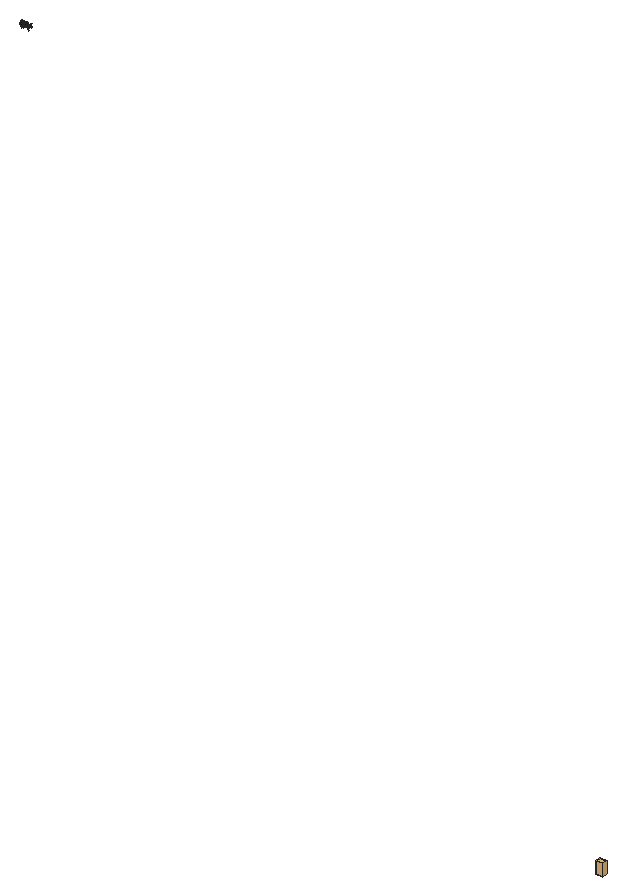
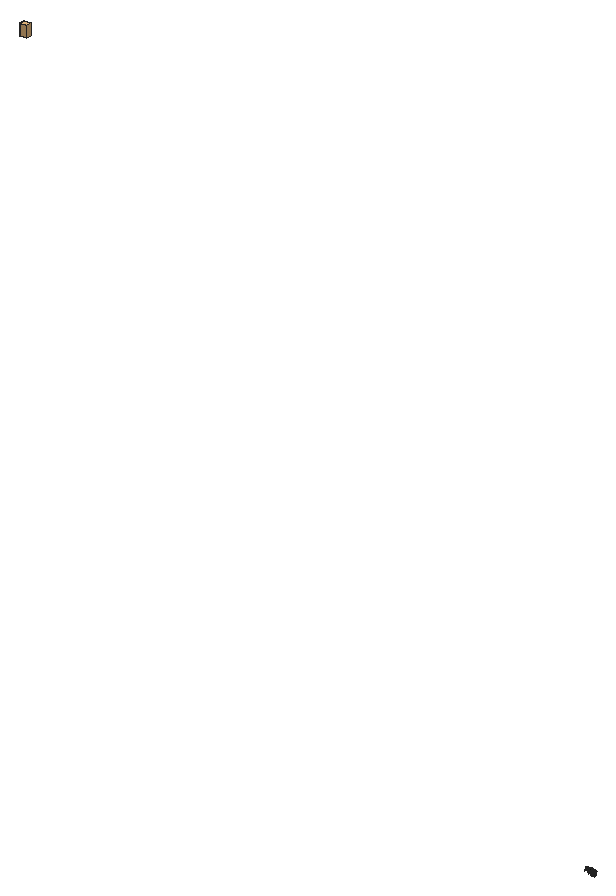
# SketchUp Ruby script. Lengths in inches.
U = 1.inch
M = Sketchup.active_model
def pt(a) = Geom::Point3d.new(a.map { |v| v * U })
def face(e, loops, mat)
  f = e.add_face(loops[0].map { |a| pt(a) })
  loops[1..].each { |l| e.add_face(l.map { |a| pt(a) }).erase! }
  f.material = f.back_material = mat if mat
  f
end
# faces: each face lists its corners as indices into pts; further lists are holes
def faces(e, pts, list, mat = nil) = list.each { |f| face(e, (f[0].is_a?(Array) ? f : [f]).map { |l| l.map { |i| pts[i] } }, mat) }
# xy, xz, yz: faces in a plane at the given z, y or x. An outline is a flat list of corners, or four numbers for a rectangle; further outlines are holes
def ring(l) = l.size == 4 ? [[l[0], l[1]], [l[2], l[1]], [l[2], l[3]], [l[0], l[3]]] : l.each_slice(2).to_a
def flat(e, list, mat, &to3) = list.each { |f| face(e, (f[0].is_a?(Array) ? f : [f]).map { |l| ring(l).map { |u, v| to3.(u, v) } }, mat) }
def xy(e, z, list, mat = nil) = flat(e, list, mat) { |x, y| [x, y, z] }
def xz(e, y, list, mat = nil) = flat(e, list, mat) { |x, z| [x, y, z] }
def yz(e, x, list, mat = nil) = flat(e, list, mat) { |y, z| [x, y, z] }
def lines(e, pts, list) = list.each { |a, b| e.add_line(pt(pts[a]), pt(pts[b])) }
# prism: a flat outline (further loops are holes) pulled along v
def prism(e, loops, v, mat = nil)
  f = face(e, loops, mat); d = Geom::Vector3d.new(v.map { |x| x * U })
  f.pushpull(f.normal.samedirection?(d) ? d.length : -d.length)
end
def box(e, o, s, mat = nil) = prism(e, [[o, [o[0] + s[0], o[1], o[2]], [o[0] + s[0], o[1] + s[1], o[2]], [o[0], o[1] + s[1], o[2]]]], [0, 0, s[2]], mat)
def at(x, y, z, deg = 0) = Geom::Transformation.translation(pt([x, y, z])) * Geom::Transformation.rotation(ORIGIN, Z_AXIS, deg.degrees)
def axes(o, x, y, z) = Geom::Transformation.new([*x, 0, *y, 0, *z, 0, *pt(o).to_a, 1])
def part(name) = M.definitions.add(name)
# library, detail: a bought-in or finely detailed component or shape, given as its bounding box
def library(name, o, s) = part(name).tap { |d| box(d.entities, o, s) }
def detail(e, o, s) = box(e.add_group.entities, o, s)
def put(e, d, t, mat = nil) = e.add_instance(d, t).tap { |i| i.material = mat if mat }
def group(e, t, mat = nil) = e.add_group.tap { |g| g.transformation = t; g.material = mat if mat }.entities
root = M.entities
M.materials.add("efeu1").color = [18, 25, 13]
M.materials.add("efeu2").color = [43, 57, 29]
c1 = part("ivyleaf_10")
p = [[0,0.5,-0.03],[-0.0625,2.02,-0.43],[-0.19,2.01,-0.46],[-0.54,1.05,-0.29],[-0.52,0.625,-0.18],[-0.83,0.76,-0.28],
  [-1.16,0.64,-0.33],[-1.15,0.33,-0.24],[-0.77,-0.39,0.02],[-0.3,-0.51,0.16],[0.04,-0.48,0.23],[-0.02,2.01,-0.4375],
  [-0.06,2.01,-0.43],[0.04,-0.49,0.23],[0.67,-0.49,0.14],[1.38,0.36,-0.2],[1.375,0.51,-0.24],[0.81,0.65,-0.19],
  [0.62,0.59,-0.15],[0.6,1.09,-0.28],[0.5,1.23,-0.31]]
faces(c1.entities,p,[[0,1,2,3,4,5,6,7,8,9,10],[11,12,0,13,14,15,16,17,18,19,20]],"efeu2")
c2 = part("ivyleaf_9")
p = [[1.54,2.16,1.25],[1.36,2.04,1.19],[-0.21,0.99,0.68],[-0.71,1.11,0.82],[-0.85,0.86,0.67],[-0.8,0.17,0.21],
  [-0.9,-0.01,0.1],[-0.67,-0.16,-0.02],[-0.08,-0.08,-0.05],[-0.03,-0.6,-0.4],[0.65,-0.88,-0.66],[0.83,-0.6,-0.49],
  [1.29,-0.42,-0.43],[1.8125,-0.07,-0.26],[1.21,0.44,0.15]]
faces(c2.entities,p,[[0,1,2,3,4,5,6,7,8,9,10,11,12,13,14]],"efeu1")
c3 = library("climbing plant",[8874.76,-5589.78,-33.625],[50.13,38.07,87.16])
put(root,c1,axes([621.93,121.28,226.16],[0.13082,-0.25494,1.16798],[0.40166,-1.09728,-0.2845],[1.12598,0.42104,-0.03422]))
put(root,c2,axes([622.5,124.66,242.44],[0.53966,1.06788,-0.68334],[-0.33052,-0.59849,-1.19629],[-1.22396,0.63246,0.02175]))
put(root,c2,axes([622.11,126.98,230.96],[-0.34371,-1.10084,0.46067],[-0.11299,-0.44722,-1.15301],[1.18798,-0.36104,0.02362]))
put(root,c1,axes([621.82,114.79,216.59],[-0.02547,0.04758,-1.24777],[0.56697,-1.11152,-0.05396],[-1.11254,-0.56754,0.00107]))
put(root,c1,axes([623.51,125.62,220.67],[-0.38394,-0.04178,-1.20552],[-1.20019,-0.11329,0.38617],[-0.12064,1.2601,-0.00525]))
put(root,c2,axes([621.81,127.83,241.53],[0.30136,-0.78689,1.13604],[0.39554,-1.06499,-0.8426],[1.32414,0.49721,-0.00686]))
put(root,c2,axes([622.67,114.96,223.21],[0.6946,-1.25849,-0.18746],[0.1308,-0.14182,1.43673],[-1.26563,-0.70533,0.0456]))
put(root,c2,axes([622.46,119.8125,213.96],[-0.05212,-1.08216,-0.44479],[0.01759,0.44446,-1.08341],[1.16988,-0.05489,-0.00353]))
put(root,c2,axes([622.64,110.83,234.17],[-0.73124,-0.71709,-0.95676],[0.6586,0.69446,-1.02385],[0.99792,-0.98378,-0.02536]))
put(root,c1,axes([623.92,130.71,215.93],[0.94267,-0.03003,0.77871],[-0.77496,0.09259,0.9417],[-0.08207,-1.2192,0.05234]))
put(root,c2,axes([622.74,126.07,231.94],[0.52099,0.99348,-0.59587],[0.2293,0.55199,1.12081],[1.13555,-0.56726,0.04706]))
put(root,c1,axes([623.71,120.03,233.7],[0.17738,-1.1205,0.34459],[0.0696,-0.33783,-1.13435],[1.17022,0.18994,0.01523]))
put(root,c2,axes([624.03,124.35,241.05],[-0.4946,0.95537,-0.5898],[0.27717,-0.52065,-1.07579],[-1.08801,-0.56694,-0.00594]))
put(root,c2,axes([624.48,124.64,228.18],[-0.48708,-0.13914,1.16323],[-1.09762,-0.38615,-0.5058],[0.40951,-1.20052,0.02787]))
put(root,c1,axes([623.02,118.5,240.74],[0.43919,0.28464,-1.10778],[0.94856,0.57241,0.52314],[0.6391,-1.04519,-0.01518]))
put(root,c1,axes([624.625,121.18,207.61],[-1.11228,-0.23607,0.54624],[-0.53634,-0.10386,-1.13702],[0.25776,-1.23481,-0.00879]))
put(root,c2,axes([623.6,132.88,214.39],[1.25204,-0.20932,0.08423],[0.08485,-0.00328,-1.26937],[0.20907,1.25487,0.01073]))
put(root,c2,axes([624.98,118.9,210.86],[-0.64118,0.35245,-0.99221],[-0.86474,0.48655,0.73165],[0.60077,1.0765,-0.00583]))
put(root,c2,axes([624.82,119.99,223.33],[-0.10094,-0.80205,1.017],[0.00799,-1.02045,-0.80398],[1.29519,-0.05621,0.08421]))
put(root,c2,axes([625.66,122.08,216.17],[0.87077,0.943,-0.26104],[-0.17566,-0.1931,-1.28355],[-0.96257,0.88831,-0.00191]))
put(root,c1,axes([625.59,123.86,235.36],[0.90257,-0.82679,0.12869],[0.09799,-0.08355,-1.224],[0.83099,0.90786,0.00455]))
put(root,c2,axes([624.79,125.24,216.72],[0.67522,-0.24603,-1.04616],[1.0708,0.0488,0.67964],[-0.09152,-1.24418,0.23353]))
put(root,c2,axes([625.66,115.16,237.83],[1.14394,-0.56801,0.34023],[-0.29925,0.16232,1.27714],[-0.59063,-1.18237,0.01188]))
put(root,c2,axes([625.33,125.91,222.91],[0.48828,0.94128,-0.71449],[0.32789,0.63481,1.06039],[1.13534,-0.58816,0.00104]))
put(root,c2,axes([626.22,123.37,227.66],[0.60308,-1.12311,-0.10996],[0.08279,-0.08031,1.27431],[-1.12544,-0.60774,0.03482]))
put(root,c2,axes([625.87,121.06,230.2],[-0.55052,0.13223,1.13004],[1.05429,-0.41265,0.5619],[0.42772,1.18734,0.06943]))
put(root,c2,axes([626.75,134.21,227.1],[-0.75708,-0.64526,0.84904],[0.65741,0.53746,0.99466],[-0.83967,1.00259,0.01323]))
put(root,c2,axes([626.33,122.01,222.71],[0.43582,-0.97376,-0.90291],[-0.36981,0.8237,-1.06683],[1.27542,0.57157,-0.0008]))
put(root,c2,axes([626.58,118.56,208.08],[0.95637,0.78651,0.07735],[0.05937,0.04958,-1.23825],[-0.78807,0.95821,0.00058]))
put(root,c2,axes([626.82,116.79,218.87],[-0.59204,-1.25495,0.25151],[-0.08075,-0.23993,-1.38729],[1.27736,-0.59683,0.02887]))
put(root,c1,axes([626.46,118.52,214.75],[1.13233,-0.03499,0.50113],[0.50126,-0.00262,-1.13281],[0.03306,1.23827,0.01177]))
put(root,c2,axes([627.52,122.18,230.47],[-0.4725,-0.58932,1.07726],[-0.63085,-0.87378,-0.75471],[1.05348,-0.78756,0.03122]))
put(root,c2,axes([626.76,129.92,236.12],[-0.49898,-0.18742,1.24288],[1.22458,0.22896,0.52615],[-0.28334,1.31958,0.08523]))
put(root,c2,axes([626.75,117.62,223.79],[0.42202,-0.97905,0.86332],[0.32596,-0.79954,-1.06605],[1.26397,0.53308,-0.01333]))
put(root,c2,axes([627.86,121.79,229.6],[0.16157,-0.24738,-1.42447],[-0.42564,1.36167,-0.28475],[1.38172,0.44839,0.07885]))
put(root,c2,axes([627.77,116.65,224.3],[0.19657,-1.35624,0.37835],[0.09699,-0.36807,-1.36978],[1.40468,0.21521,0.04163]))
put(root,c2,axes([628.09,128.66,243.78],[1.06349,-0.69891,-0.48286],[-0.40497,0.26298,-1.27259],[0.74675,1.13798,-0.00247]))
put(root,c2,axes([627.87,121.77,231.24],[1.26844,-0.32266,0.13001],[0.12759,-0.0258,-1.30882],[0.32363,1.27483,0.00642]))
put(root,c2,axes([628.49,115.81,237.61],[-0.53631,-0.87006,-1.01848],[0.48943,0.89395,-1.02139],[1.2469,-0.72512,-0.03715]))
put(root,c2,axes([630.52,122.6,240.92],[-1.01134,-0.30167,1.02001],[-0.98447,-0.26753,-1.05522],[0.40281,-1.41126,-0.018]))
put(root,c2,axes([628.68,119.51,215.12],[-0.05844,-0.09754,1.41171],[0.88591,-1.10428,-0.03962],[1.10345,0.88142,0.10658]))
put(root,c1,axes([630.4,123.07,211.1],[-0.44298,-1.11351,0.31678],[-0.12316,-0.29193,-1.19837],[1.15112,-0.45974,-0.00631]))
put(root,c1,axes([630.14,129.3,240.63],[0.19549,-0.31815,1.19268],[0.61951,-1.01917,-0.37341],[1.06767,0.64962,-0.00171]))
put(root,c2,axes([629.84,117.59,242.41],[0.24488,0.03114,-1.3683],[1.36114,0.13996,0.24678],[0.14326,-1.38298,-0.00584]))
put(root,c2,axes([630.65,119.62,232.26],[-0.59727,-1.18153,-0.5536],[0.21892,0.50947,-1.32353],[1.28629,-0.63533,-0.0318]))
put(root,c2,axes([631.52,110.98,227.94],[0.70827,1.03381,-0.84738],[-0.53116,-0.66236,-1.25205],[-1.22666,0.88373,0.05288]))
put(root,c2,axes([630.64,123.7,221.57],[0.31645,-0.33114,1.15761],[0.93246,-0.68983,-0.45223],[0.76174,0.98201,0.07268]))
put(root,c1,axes([631.13,120.36,236.35],[-0.48912,0.33884,-1.09093],[0.93775,-0.5586,-0.59394],[-0.65235,-1.05704,-0.03583]))
put(root,c2,axes([631.33,111.5,224.18],[-0.0334,-0.29208,-1.48571],[0.78784,1.26571,-0.26654],[1.29304,-0.77874,0.12402]))
put(root,c2,axes([631.82,125.47,213.79],[-0.08103,0.94529,0.90342],[0.0495,-0.90228,0.94854],[1.30663,0.0928,0.02009]))
put(root,c2,axes([631.21,119.63,229.59],[0.39516,0.11839,-1.36777],[1.22322,0.61585,0.4067],[0.62332,-1.28362,0.06898]))
put(root,c2,axes([631.89,124.52,213.03],[0.07708,-0.07267,1.29043],[1.04205,-0.76125,-0.10511],[0.7646,1.04481,0.01317]))
put(root,c2,axes([632.12,118.89,229.34],[0.35838,-0.58247,1.2473],[0.58292,-1.10341,-0.68276],[1.24709,0.68314,-0.0393]))
put(root,c2,axes([632.89,125.73,238.55],[-0.61157,-0.25419,-1.10463],[1.02529,0.41114,-0.66226],[0.48332,-1.19381,0.00713]))
put(root,c2,axes([633.72,124.87,236.49],[0.94419,-0.67248,-0.66365],[0.53795,-0.38867,1.15919],[-0.77671,-1.08668,-0.00391]))
put(root,c1,axes([633.59,129.45,222],[0.34574,0.02935,1.20866],[1.16247,0.33738,-0.34073],[-0.33224,1.21102,0.06563]))
put(root,c1,axes([634.79,127.62,237.97],[0.50318,0.5879,-0.99875],[0.53716,0.8465,0.7689],[1.02693,-0.73084,0.08718]))
put(root,c2,axes([634.93,120.11,224.31],[0.89009,0.57239,0.75218],[0.63103,0.40938,-1.05825],[-0.70372,1.09108,0.00245]))
put(root,c2,axes([635.91,118.98,234.96],[-0.19894,0.28865,-1.40935],[-0.86133,1.11567,0.35008],[1.15226,0.88381,0.01837]))
put(root,c2,axes([634.82,124.58,242.98],[-0.089,-0.06093,-1.33903],[1.24725,0.4878,-0.1051],[0.49099,-1.25019,0.02425]))
put(root,c2,axes([635.47,128.01,234.09],[0.18009,1.12591,-0.5523],[0.0454,0.55174,1.13959],[1.25325,-0.18178,0.03808]))
put(root,c2,axes([635.58,111.67,209.23],[0.7311,-0.66925,-0.85109],[0.742,-0.43817,0.98194],[-0.78847,-1.03289,0.1349]))
put(root,c2,axes([636.34,129.41,229.71],[-0.74973,-0.31351,-0.98532],[0.90235,0.39589,-0.81256],[0.50487,-1.17312,-0.01089]))
put(root,c2,axes([636.23,129.96,220.84],[0.69071,-1.13036,0.40509],[0.23943,-0.32829,-1.32431],[1.17664,0.73035,0.03168]))
put(root,c2,axes([637.14,119.93,231.22],[1.15296,-0.35702,0.50322],[-0.46653,0.1935,1.2062],[-0.40378,-1.24302,0.04324]))
put(root,c2,axes([638.64,116.125,226.7],[-0.89367,-1.02299,-0.11982],[-0.07913,-0.08998,1.35836],[-1.02693,0.89717,-0.0004]))
put(root,c2,axes([639.26,116.27,234.54],[-1.229,-0.12499,-0.3778],[-0.37609,-0.03593,1.23534],[-0.13003,1.28525,-0.0022]))
put(root,c2,axes([638.15,130.68,214.375],[-0.05709,-0.07814,1.27897],[1.17685,0.50322,0.08328],[-0.50686,1.1772,0.0493]))
put(root,c2,axes([638.2,127.49,222.125],[-0.07296,-0.1971,-1.26169],[1.24796,0.25693,-0.11231],[0.27074,-1.2374,0.17765]))
put(root,c2,axes([639.6,124.35,235.54],[0.2418,-0.56988,-1.33838],[-0.4991,1.24189,-0.61896],[1.36636,0.55448,0.01076]))
put(root,c2,axes([640.02,122.5,223.41],[-1.09177,-0.34123,-0.57667],[0.55908,0.1438,-1.14355],[0.36935,-1.22631,0.02637]))
put(root,c2,axes([639.22,118.66,234.9],[-0.19391,0.01017,1.3096],[1.21268,-0.49851,0.18343],[0.49453,1.22643,0.0637]))
put(root,c2,axes([641.98,118.66,226.54],[-1.2554,-0.07984,-0.57226],[-0.57144,-0.03104,1.25792],[-0.08552,1.37932,-0.00482]))
put(root,c2,axes([642.24,126.03,208.36],[-0.63205,-0.11207,-1.16735],[-1.13183,-0.28881,0.64054],[-0.30696,1.29567,0.04181]))
put(root,c2,axes([640.77,122.45,211.16],[0.08947,-0.06594,-1.32036],[0.6436,1.15813,-0.01423],[1.15476,-0.64037,0.11023]))
put(root,c2,axes([640.82,120.89,242.03],[1.20042,-0.60886,0.02526],[0.02425,-0.00805,-1.34599],[0.6089,1.20066,0.00379]))
put(root,c2,axes([642.48,121.62,218.52],[-0.31324,-1.2984,-0.05208],[0.01375,0.05026,-1.33564],[1.29937,-0.31354,0.00158]))
put(root,c2,axes([642.47,117.7,228.64],[1.22706,-0.79712,0.04283],[0.03642,-0.02257,-1.46324],[0.79744,1.2276,0.00091]))
put(root,c2,axes([644.12,116.875,212.68],[-0.04093,-0.16407,-1.34851],[-0.31019,-1.31235,0.16909],[-1.32256,0.31287,0.00207]))
put(root,c2,axes([642.65,120.98,221.08],[-0.00705,0.00792,-1.38544],[0.90601,1.04818,0.00138],[1.04816,-0.90598,-0.01051]))
put(root,c2,axes([643.86,118.68,225.82],[-0.16155,0.6613,-1.1569],[-0.29877,1.11773,0.68063],[1.29865,0.33941,0.01267]))
put(root,c2,axes([645.4,116.07,229.03],[-0.25824,0.93084,0.99709],[0.26686,-0.96071,0.966],[1.3377,0.37135,-0.00023]))
put(root,c2,axes([646.23,122.48,230.57],[0.52907,-1.03457,-0.70881],[0.35943,-0.61195,1.16146],[-1.20148,-0.63864,0.03533]))
put(root,c2,axes([646.57,122.82,218.07],[0.26194,0.35802,1.28119],[0.79477,1.005,-0.44333],[-1.06676,0.83667,-0.01571]))
put(root,c2,axes([646.2,115.96,242.11],[-0.09876,-0.42717,-1.39353],[0.57834,1.27058,-0.43047],[1.33788,-0.58078,0.08322]))
put(root,c2,axes([647.62,114.8,229.58],[0.15235,0.2178,-1.29973],[0.80162,1.02318,0.26542],[1.04601,-0.81584,-0.0141]))
put(root,c2,axes([648.64,119.47,230.9],[0.06569,-1.40203,-0.1705],[-0.02306,0.16959,-1.40349],[1.41217,0.06798,-0.01499]))
put(root,c2,axes([648.89,121.8,212.61],[-0.03308,-0.55754,-1.23541],[0.26565,1.20914,-0.5528],[1.32911,-0.25554,0.07974]))
put(root,c2,axes([652.0625,118.16,238.12],[-0.69153,0.17175,-1.23057],[-1.20519,0.24979,0.71213],[0.30218,1.38929,0.02409]))
put(root,c2,axes([652.29,108.16,215.82],[0.98842,0.49753,-0.81601],[-0.73835,-0.34785,-1.10645],[-0.60683,1.23363,0.01712]))
put(root,c2,axes([652.74,126.96,242.66],[1.17327,-0.61221,0.19114],[0.16531,-0.09636,-1.32336],[0.61969,1.18482,-0.00887]))
put(root,c2,axes([653.67,124.72,219.52],[0.51357,-1.27302,-0.3118],[-0.12494,0.28581,-1.37268],[1.30468,0.52848,-0.00871]))
put(root,c2,axes([654.47,115.21,237.12],[0.16622,-0.21391,-1.36498],[-0.37324,1.31675,-0.2518],[1.33026,0.39618,0.0999]))
put(root,c2,axes([655.58,126.64,242.98],[-0.02655,-0.17538,-1.33524],[0.03217,1.33503,-0.17599],[1.34632,-0.03536,-0.02213]))
put(root,c2,axes([657.5625,131.72,223.05],[1.07614,-0.7505,-0.53072],[-0.43489,0.30419,-1.312],[0.80981,1.16069,0.00068]))
put(root,c2,axes([658.47,124.1875,238.8],[0.21133,0.92172,0.96386],[0.17671,0.94793,-0.94523],[-1.32188,0.27407,0.02774]))
put(root,c2,axes([658.36,125.61,235.9375],[-0.61288,-0.16285,-1.20292],[1.18683,0.20255,-0.6321],[0.25488,-1.33477,0.05084]))
put(root,c2,axes([658.85,121.46,240.125],[0.89382,0.83853,0.7263],[0.52407,0.50291,-1.22556],[-0.97775,1.03611,0.00707]))
put(root,c2,axes([658.13,128.78,229.98],[0.6174,0.11947,-1.3361],[1.33091,0.12929,0.62656],[0.16768,-1.46616,-0.05362]))
put(root,c2,axes([660.39,107.52,228.48],[-0.25616,1.26819,0.69926],[-0.21485,0.66898,-1.29197],[-1.43217,-0.32719,0.06875]))
put(root,c2,axes([660.95,117.69,228.97],[-0.36189,0.50533,-1.32946],[-0.82722,1.04113,0.62091],[1.15695,0.90248,0.0281]))
put(root,c2,axes([662.82,110.3,227.54],[0.23656,-0.37698,1.31168],[-0.70374,1.10692,0.44505],[-1.16935,-0.74243,-0.00248]))
put(root,c2,axes([662.07,126.51,223.73],[-0.27203,-1.31142,0.28322],[-0.06502,-0.27576,-1.33931],[1.34008,-0.27959,-0.00749]))
put(root,c2,axes([662.78,125.52,242.83],[-0.93421,0.83294,-0.57523],[0.38154,-0.43529,-1.24995],[-0.93761,-1.00705,0.06451]))
put(root,c2,axes([662.76,112.21,240.93],[0.32043,1.26118,0.47547],[-0.18067,-0.44412,1.29978],[1.33566,-0.36263,0.06175]))
put(root,c2,axes([663.78,106.28,242.1],[0.89126,-1.17957,0.11251],[0.07574,-0.08379,-1.47839],[1.1825,0.89442,0.00989]))
put(root,c2,axes([664.89,122.21,236.69],[-0.04719,-0.32931,-1.41762],[0.00548,1.41831,-0.32966],[1.45535,-0.01602,-0.04472]))
put(root,c2,axes([665.63,126.05,229.1],[0.76157,0.31198,1.10789],[-1.01835,-0.43645,0.82292],[0.53639,-1.27158,-0.01063]))
put(root,c2,axes([665.78,123.04,219.67],[-1.01171,0.44939,-0.82201],[0.72619,-0.38816,-1.10598],[-0.59187,-1.24442,0.04813]))
put(root,c2,axes([665.47,106.61,236.14],[1.11529,-0.51033,-0.84508],[-0.76489,0.3594,-1.22648],[0.62414,1.35236,0.00704]))
put(root,c2,axes([665,126.14,224.91],[-0.13265,0.11052,1.36883],[0.74736,-1.14791,0.16511],[1.15211,0.75736,0.0505]))
put(root,c2,axes([666.34,123.79,237.2],[1.22337,-0.35894,-0.52729],[0.5115,-0.12937,1.27481],[-0.3811,-1.32587,0.01836]))
put(root,c2,axes([666.95,121.08,242.33],[0.57099,1.13163,-0.73366],[0.29066,0.67472,1.26694],[1.31695,-0.63955,0.03846]))
put(root,c2,axes([672.51,121.25,209.41],[0.48837,-0.75388,-1.08236],[-0.54341,0.93668,-0.8976],[1.20189,0.72982,0.03397]))
put(root,c2,axes([672.76,108.79,226.11],[-0.71138,-0.40007,1.16251],[0.98535,0.61767,0.81554],[-0.73523,1.21489,-0.03181]))
put(root,c2,axes([674.9,122.63,233.66],[0.08799,-0.12986,-1.44929],[-0.96307,1.08321,-0.15553],[1.09077,0.96687,-0.0204]))
put(root,c2,axes([677.34,109.95,239.72],[-0.42017,0.08164,1.37651],[-1.35374,0.24936,-0.42801],[-0.26235,-1.41744,0.00398]))
put(root,c2,axes([683.87,118.8,235.53],[0.81365,-1.04801,-0.70223],[-0.42789,0.55682,-1.32678],[1.18675,0.9193,0.00308]))
put(root,c2,axes([685.98,123.85,229.55],[-0.76576,-1.15652,0.4312],[0.237,0.36023,1.38706],[-1.21132,0.8016,-0.00121]))
put(root,c2,axes([688.94,113.3,222.15],[-0.71028,1.21898,-0.38659],[0.19897,-0.33149,-1.41081],[-1.26324,-0.73761,-0.00485]))
put(root,c2,axes([687.88,127,241.52],[0.36998,1.09419,-0.91304],[0.27667,0.87021,1.15497],[1.39798,-0.4618,0.01306]))
put(root,c2,axes([690.02,108.27,237.84],[0.9385,-1.11849,-0.28538],[0.19422,-0.20956,1.46],[-1.13787,-0.95829,0.01382]))
put(root,c2,axes([690.72,105.8,207.34],[-0.06727,0.38205,1.42749],[0.25587,-1.40438,0.38792],[1.45541,0.26456,-0.00222]))
put(root,c2,axes([696.3125,126.94,223.5],[-1.3388,0.25344,-0.64629],[-0.63267,0.13247,1.36253],[0.28575,1.48072,-0.01127]))
put(root,c2,axes([698.55,112.92,237.42],[1.29853,0.47011,-0.56943],[-0.53728,-0.18869,-1.381],[-0.50653,1.40529,0.00506]))
put(root,c3,at(662.17,-85.8125,266.59))
